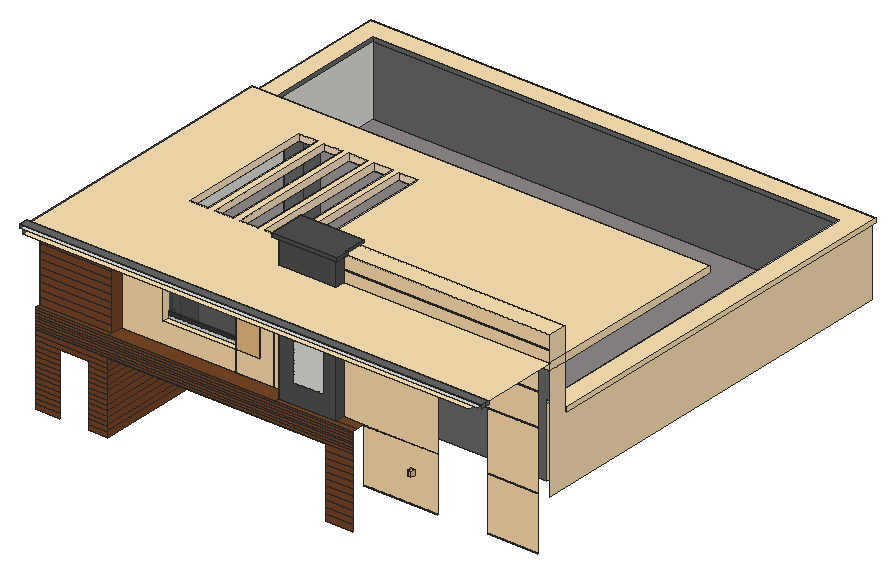
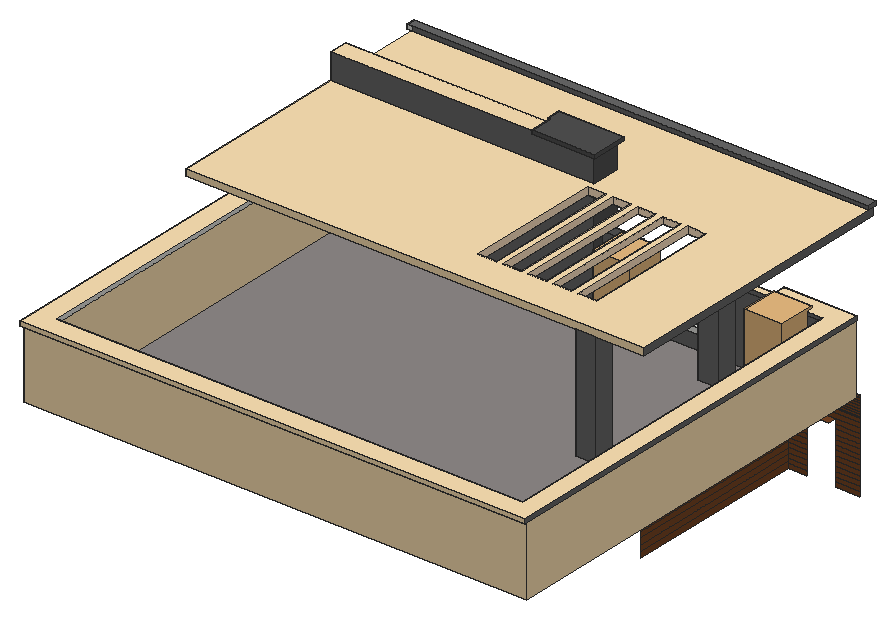
# SketchUp Ruby script. Lengths in inches.
U = 1.inch
M = Sketchup.active_model
def pt(a) = Geom::Point3d.new(a.map { |v| v * U })
def face(e, loops, mat)
  f = e.add_face(loops[0].map { |a| pt(a) })
  loops[1..].each { |l| e.add_face(l.map { |a| pt(a) }).erase! }
  f.material = f.back_material = mat if mat
  f
end
# faces: each face lists its corners as indices into pts; further lists are holes
def faces(e, pts, list, mat = nil) = list.each { |f| face(e, (f[0].is_a?(Array) ? f : [f]).map { |l| l.map { |i| pts[i] } }, mat) }
# xy, xz, yz: faces in a plane at the given z, y or x. An outline is a flat list of corners, or four numbers for a rectangle; further outlines are holes
def ring(l) = l.size == 4 ? [[l[0], l[1]], [l[2], l[1]], [l[2], l[3]], [l[0], l[3]]] : l.each_slice(2).to_a
def flat(e, list, mat, &to3) = list.each { |f| face(e, (f[0].is_a?(Array) ? f : [f]).map { |l| ring(l).map { |u, v| to3.(u, v) } }, mat) }
def xy(e, z, list, mat = nil) = flat(e, list, mat) { |x, y| [x, y, z] }
def xz(e, y, list, mat = nil) = flat(e, list, mat) { |x, z| [x, y, z] }
def yz(e, x, list, mat = nil) = flat(e, list, mat) { |y, z| [x, y, z] }
def lines(e, pts, list) = list.each { |a, b| e.add_line(pt(pts[a]), pt(pts[b])) }
# prism: a flat outline (further loops are holes) pulled along v
def prism(e, loops, v, mat = nil)
  f = face(e, loops, mat); d = Geom::Vector3d.new(v.map { |x| x * U })
  f.pushpull(f.normal.samedirection?(d) ? d.length : -d.length)
end
def box(e, o, s, mat = nil) = prism(e, [[o, [o[0] + s[0], o[1], o[2]], [o[0] + s[0], o[1] + s[1], o[2]], [o[0], o[1] + s[1], o[2]]]], [0, 0, s[2]], mat)
def at(x, y, z, deg = 0) = Geom::Transformation.translation(pt([x, y, z])) * Geom::Transformation.rotation(ORIGIN, Z_AXIS, deg.degrees)
def axes(o, x, y, z) = Geom::Transformation.new([*x, 0, *y, 0, *z, 0, *pt(o).to_a, 1])
def part(name) = M.definitions.add(name)
# library, detail: a bought-in or finely detailed component or shape, given as its bounding box
def library(name, o, s) = part(name).tap { |d| box(d.entities, o, s) }
def detail(e, o, s) = box(e.add_group.entities, o, s)
def put(e, d, t, mat = nil) = e.add_instance(d, t).tap { |i| i.material = mat if mat }
def group(e, t, mat = nil) = e.add_group.tap { |g| g.transformation = t; g.material = mat if mat }.entities
root = M.entities
M.materials.add("KORKULUK CAMI").color = [72, 76, 73]
M.materials["KORKULUK CAMI"].alpha = 0.5
M.materials.add("KORKULUK PROFİL").color = [58, 58, 58]
M.materials.add("[0012_Bisque]").color = [255, 228, 196]
M.materials.add("[0032_Moccasin]").color = [255, 228, 181]
M.materials.add("[0033_NavajoWhite]").color = [255, 222, 173]
M.materials.add("[0134_DimGray]").color = [105, 105, 105]
M.materials.add("[0135_DarkGray]").color = [81, 81, 81]
M.materials.add("[Stone Marble]").color = [143, 138, 136]
M.materials.add("[Wood Veneer 01]").color = [120, 70, 37]
c1 = library("Lamp Wall Outdoor 94-02",[-1.89,-4.65,-3.17],[3.78,4.65,6.35])
c2 = library("plant",[-22.43,-22.29,0],[44.86,44.58,89.56])
c3 = part("CAM KORKULUK")
g1 = group(c3.entities,at(15.11,0,0))
g2 = group(g1,at(31.92,0.79,0),"KORKULUK CAMI")
xy(g2,3.9375,[[-46.24,0,19.11,0.39],[-46.24,0.39,-45.85,7.09],[18.72,0.39,19.11,7.09]])
xy(g2,35.43,[[-46.24,0,19.11,0.39],[-46.24,0.39,-45.85,7.09],[18.72,0.39,19.11,7.09]])
xz(g2,0,[[-46.24,3.9375,19.11,35.43]])
xz(g2,0.39,[[-46.24,3.9375,-45.85,35.43],[-45.85,3.9375,18.72,35.43],[18.72,3.9375,19.11,35.43]])
xz(g2,7.09,[[-46.24,3.9375,-45.85,35.43],[18.72,3.9375,19.11,35.43]])
yz(g2,-46.24,[[0,3.9375,0.39,35.43],[0.39,3.9375,7.09,35.43]])
yz(g2,-45.85,[[0.39,3.9375,7.09,35.43]])
yz(g2,18.72,[[0.39,3.9375,7.09,35.43]])
yz(g2,19.11,[[0,3.9375,0.39,35.43],[0.39,3.9375,7.09,35.43]])
g3 = group(g1,at(95.77,0,0),"KORKULUK PROFİL")
prism(g3,[[[-110.875,0,0],[-110.875,7.875,0],[-108.91,7.875,0],[-108.91,1.97,0],[-45.91,1.97,0],[-45.91,7.875,0],[-43.95,7.875,0],[-43.95,0,0]]],[0,0,3.9375])
g4 = group(g1,at(95.77,0.39,35.43))
prism(g4,[[[-110.48,0,0],[-110.48,7.48,0],[-109.3,7.48,0],[-109.3,1.18,0],[-45.52,1.18,0],[-45.52,7.48,0],[-44.34,7.48,0],[-44.34,0,0]]],[0,0,0.79],"KORKULUK PROFİL")
g5 = group(c3.entities,at(0,0,-7.875))
box(g5,[0,0,0],[66.93,7.875,7.875])
c4 = library("Tlon Light 950 Ceiling 152 008",[-18.7,-18.7,-3.78],[37.4,37.4,3.56])
xy(root,219.625,[[1583.17,528.0625,1636.42,600.9375],[1636.42,528.0625,1668.92,600.9375]])
xy(root,221.7,[[1460.375,309.8125,1494.3,320.75]],"[Wood Veneer 01]")
xy(root,233,[[1518,309.8125,1518,528.0625,1777.8125,528.0625,1777.8125,330.25,1674.625,330.25,1674.625,319.48,1681.5,319.48,1681.5,319.875,1688.38,319.875,1688.38,319.48,1695.26,319.48,1695.26,319.875,1702.14,319.875,1702.14,319.48,1709.02,319.48,1709.02,319.875,1715.9,319.875,1715.9,319.48,1722.78,319.48,1722.78,319.875,1729.66,319.875,1729.66,319.48,1736.54,319.48,1736.54,319.875,1743.42,319.875,1743.42,319.48,1750.3,319.48,1750.3,319.875,1757.18,319.875,1757.18,319.48,1764.05,319.48,1764.05,319.875,1770.93,319.875,1770.93,319.48,1777.8125,319.48,1777.8125,309.8125]],"[Wood Veneer 01]")
xy(root,257,[[[1453.13,337.57,1717.17,337.57,1717.17,349.32,2009.5,349.32,2009.5,785.68,1453.13,785.68],[1542.22,541.15,1566.53,565.47],[1542.22,357.72,1566.53,382.03]]],"[Stone Marble]")
xy(root,257,[[1431.3125,309.8125,1518,315.75],[1518,309.8125,1717.17,329.6875],[1717.17,309.8125,1809.4375,315.75],[1784.8125,315.75,1809.4375,327.3125]],"[Wood Veneer 01]")
xy(root,281.625,[[1567.79,329.6875,1682.98,337.57]],"[0032_Moccasin]")
xy(root,326.75,[[1897.5625,327.3125,1957.25,348.375]])
xy(root,339.3125,[[1430.8125,315.25,1518,315.75],[1430.8125,315.75,1431.3125,809.9375],[1518,329.1875,1567.79,329.6875],[2031.3125,349.32,2033.75,807.5],[1431.3125,807.5,2033.75,809.9375]])
xy(root,339.3125,[[1677.98,324.6875,1717.17,329.6875],[1677.98,329.6875,1682.98,337.57]],"[0135_DarkGray]")
xy(root,344.3125,[[1430.8125,315.25,1518,315.25,1518,329.1875,1567.79,329.1875,1567.79,337.57,1453.13,337.57,1453.13,785.68,2009.5,785.68,2009.5,349.32,2033.75,349.32,2033.75,809.9375,1430.8125,809.9375]],"[0032_Moccasin]")
xy(root,344.3125,[[1677.98,324.6875,1717.17,337.57]],"[0135_DarkGray]")
xy(root,392.3125,[[2017.03,327.3125,2031.3125,327.5],[1542.22,357.72,1566.53,382.03],[1542.22,541.15,1566.53,565.47]])
xy(root,392.3125,[[1485.22,541.15,1542.22,565.47],[1566.53,541.15,2031.3125,565.47]],"[0012_Bisque]")
xy(root,392.3125,[[[1485.22,223.9375,1485.22,541.15,2031.3125,541.15,2031.3125,327.5,2017.03,327.5,2017.03,223.9375],[1576.06,358.48,1598.12,522.05],[1605.9,358.48,1627.96,522.05],[1635.75,358.48,1657.81,522.05],[1665.59,358.48,1687.65,522.05],[1695.43,358.48,1717.5,522.05],[1542.22,357.72,1566.53,382.03]]],"[0032_Moccasin]")
xy(root,400.3125,[[1485.22,218.9375,2031.3125,223.9375]])
xy(root,400.3125,[[[1485.22,228.9375,2031.3125,565.47],[1576.06,358.48,1598.12,522.05],[1605.9,358.48,1627.96,522.05],[1635.75,358.48,1657.81,522.05],[1665.59,358.48,1687.65,522.05],[1695.43,358.48,1717.5,522.05]]],"[0032_Moccasin]")
xy(root,405.3125,[[1485.22,218.9375,2036.3125,228.9375]],"[0134_DimGray]")
xy(root,430.75,[[1717.17,315.75,1717.17,349.32,1786.8125,349.32,1786.8125,327.3125,1784.8125,327.3125,1784.8125,315.75],[1784.8125,315.75,1789.8125,327.3125],[1786.8125,327.3125,1789.8125,327.5]])
xy(root,430.75,[[1789.8125,327.3125,2031.3125,327.3125,2031.3125,349.32,1786.8125,349.32,1786.8125,327.5,1789.8125,327.5]],"[0032_Moccasin]")
xy(root,430.75,[[1712.17,310.75,1789.8125,315.75],[1712.17,315.75,1717.17,354.32],[1717.17,349.32,1786.8125,354.32]],"[0135_DarkGray]")
xy(root,434.9375,[[1712.17,310.75,1789.8125,310.75,1789.8125,327.5,1786.8125,327.5,1786.8125,354.32,1712.17,354.32]],"[0135_DarkGray]")
xz(root,228.9375,[[2031.3125,400.3125,2036.3125,405.3125]])
xz(root,228.9375,[[1485.22,400.3125,2031.3125,405.3125]],"[0134_DimGray]")
xz(root,309.8125,[[1431.3125,148.25,1460.375,153.9],[1494.3,148.25,1518,153.9],[1777.8125,150.13,1809.4375,157.67],[1431.3125,153.9,1460.375,159.55],[1494.3,153.9,1518,159.55],
  [1777.8125,157.67,1809.4375,165.2],[1431.3125,159.55,1460.375,165.2],[1494.3,159.55,1518,165.2],[1431.3125,165.2,1460.375,170.85],[1494.3,165.2,1518,170.85],
  [1777.8125,165.2,1809.4375,172.73],[1431.3125,170.85,1460.375,176.5],[1494.3,170.85,1518,176.5],[1777.8125,172.73,1809.4375,180.27],[1431.3125,176.5,1460.375,182.15],
  [1494.3,176.5,1518,182.15],[1777.8125,180.27,1809.4375,187.8],[1431.3125,182.15,1460.375,187.8],[1494.3,182.15,1518,187.8],[1431.3125,187.8,1460.375,193.45],
  [1494.3,187.8,1518,193.45],[1777.8125,187.8,1809.4375,195.33],[1431.3125,193.45,1460.375,199.1],[1494.3,193.45,1518,199.1],[1777.8125,195.33,1809.4375,202.87],
  [1431.3125,199.1,1460.375,204.75],[1494.3,199.1,1518,204.75],[1777.8125,202.87,1809.4375,210.4],[1431.3125,204.75,1460.375,210.4],[1494.3,204.75,1518,210.4],
  [1431.3125,210.4,1460.375,216.05],[1494.3,210.4,1518,216.05],[1777.8125,210.4,1809.4375,217.93],[1431.3125,216.05,1460.375,221.7],[1494.3,216.05,1518,221.7],
  [1777.8125,217.93,1809.4375,225.47],[1431.3125,221.7,1518,227.35],[1777.8125,225.47,1809.4375,225.47,1809.4375,233.625,1431.3125,233.625,1431.3125,233,1777.8125,233],[1431.3125,227.35,1518,233],[1431.3125,233.625,1809.4375,236.55],
  [1431.3125,236.55,1809.4375,239.47],[1431.3125,239.47,1809.4375,242.39],[1431.3125,242.39,1809.4375,245.3125],[1431.3125,245.3125,1809.4375,248.23],[1431.3125,248.23,1809.4375,251.16],
  [1431.3125,251.16,1809.4375,254.08],[1431.3125,254.08,1809.4375,257]],"[Wood Veneer 01]")
xz(root,310.75,[[1712.17,430.75,1789.8125,434.9375]],"[0135_DarkGray]")
xz(root,315.25,[[1430.8125,339.3125,1518,344.3125]],"[0135_DarkGray]")
xz(root,315.75,[[1734.84,280.12,1768.77,347.56]])
xz(root,315.75,[[[1717.17,257,1784.8125,430.75],[1734.84,280.12,1768.77,347.56]]],"[0135_DarkGray]")
xz(root,315.75,[[1431.3125,257,1518,265.23],[1431.3125,265.23,1518,273.46],[1431.3125,273.46,1518,281.69],[1431.3125,281.69,1518,289.92],[1431.3125,289.92,1518,298.16],
  [1431.3125,298.16,1518,306.39],[1431.3125,306.39,1518,314.62],[1431.3125,314.62,1518,322.85],[1431.3125,322.85,1518,331.08],[1431.3125,331.08,1518,339.3125]],"[Wood Veneer 01]")
xz(root,324.6875,[[1677.98,339.3125,1717.17,344.3125]],"[0135_DarkGray]")
xz(root,327.3125,[[1809.4375,192.7,1897.5625,255.9375],[1957.25,192.7,2017.03,255.9375],[1809.4375,256.9375,1897.5625,256.9375,1897.5625,325.75,1784.8125,325.75,1784.8125,257,1809.4375,257],[1957.25,256.9375,2017.03,325.75],[1784.8125,326.75,2017.03,364.83],
  [1784.8125,365.83,2017.03,365.83,2017.03,392.3125,2031.3125,392.3125,2031.3125,413.25,1784.8125,413.25],[1784.8125,414.25,2031.3125,430.75]],"[0033_NavajoWhite]")
xz(root,327.3125,[[1809.4375,191.7,1897.5625,192.7],[1957.25,191.7,2017.03,192.7],[1809.4375,255.9375,1897.5625,256.9375],[1957.25,255.9375,2017.03,256.9375],[1784.8125,325.75,1897.5625,326.75],
  [1957.25,325.75,2017.03,326.75],[1784.8125,364.83,2017.03,365.83],[1784.8125,413.25,2031.3125,414.25]],"[0135_DarkGray]")
xz(root,327.5,[[1786.8125,430.75,1789.8125,434.9375]])
xz(root,329.1875,[[1518,339.3125,1567.79,344.3125]],"[0135_DarkGray]")
xz(root,329.6875,[[1518,257,1717.17,257,1717.17,339.3125,1682.98,339.3125,1682.98,281.625,1567.79,281.625,1567.79,339.3125,1518,339.3125]],"[0033_NavajoWhite]")
xz(root,337.57,[[1453.13,257,1453.13,339.3125,1567.79,339.3125,1567.79,281.625,1682.98,281.625,1682.98,339.3125,1677.98,339.3125,1677.98,344.3125,1717.17,344.3125,1717.17,257],[1453.13,339.3125,1567.79,344.3125]],"[0134_DimGray]")
xz(root,349.32,[[2031.3125,339.3125,2033.75,344.3125]])
xz(root,349.32,[[1717.17,257,1717.17,430.75,2031.3125,430.75,2031.3125,344.3125,2009.5,344.3125,2009.5,257]],"[0134_DimGray]")
xz(root,354.32,[[1712.17,430.75,1786.8125,434.9375]],"[0135_DarkGray]")
xz(root,357.72,[[1542.22,257,1566.53,392.3125]],"[0134_DimGray]")
xz(root,358.48,[[1576.06,392.3125,1598.12,400.3125],[1605.9,392.3125,1627.96,400.3125],[1635.75,392.3125,1657.81,400.3125],[1665.59,392.3125,1687.65,400.3125],[1695.43,392.3125,1717.5,400.3125]],"[0012_Bisque]")
xz(root,382.03,[[1542.22,257,1566.53,392.3125]],"[0134_DimGray]")
xz(root,522.05,[[1576.06,392.3125,1598.12,400.3125],[1605.9,392.3125,1627.96,400.3125],[1635.75,392.3125,1657.81,400.3125],[1665.59,392.3125,1687.65,400.3125],[1695.43,392.3125,1717.5,400.3125]],"[0012_Bisque]")
xz(root,541.15,[[1542.22,257,1566.53,392.3125]],"[0134_DimGray]")
xz(root,565.47,[[1485.22,392.3125,2031.3125,400.3125]],"[0032_Moccasin]")
xz(root,565.47,[[1542.22,257,1566.53,392.3125]],"[0134_DimGray]")
xz(root,785.68,[[1453.13,257,2009.5,339.3125],[1453.13,339.3125,2009.5,344.3125]],"[0134_DimGray]")
xz(root,807.5,[[1431.3125,257,2031.3125,339.3125]],"[0032_Moccasin]")
xz(root,809.9375,[[1430.8125,339.3125,2033.75,344.3125]],"[0032_Moccasin]")
yz(root,1430.8125,[[315.25,339.3125,809.9375,344.3125]],"[0134_DimGray]")
yz(root,1431.3125,[[315.75,257,807.5,339.3125]],"[0032_Moccasin]")
yz(root,1453.13,[[337.57,257,785.68,339.3125]])
yz(root,1453.13,[[337.57,339.3125,785.68,344.3125]],"[0134_DimGray]")
yz(root,1485.22,[[223.9375,392.3125,565.47,400.3125],[218.9375,400.3125,228.9375,405.3125]],"[0134_DimGray]")
yz(root,1518,[[315.25,339.3125,329.1875,344.3125]],"[0135_DarkGray]")
yz(root,1518,[[309.8125,148.2,528.0625,155.27],[309.8125,155.27,528.0625,162.33],[309.8125,162.33,528.0625,169.4],[309.8125,169.4,528.0625,176.47],[309.8125,176.47,528.0625,183.53],
  [309.8125,183.53,528.0625,190.6],[309.8125,190.6,528.0625,197.67],[309.8125,197.67,528.0625,204.73],[309.8125,204.73,528.0625,211.8],[309.8125,211.8,528.0625,218.87],
  [309.8125,218.87,528.0625,225.93],[309.8125,225.93,528.0625,233],[315.75,257,329.6875,339.3125]],"[Wood Veneer 01]")
yz(root,1542.22,[[357.72,257,382.03,392.3125],[541.15,257,565.47,392.3125]],"[0134_DimGray]")
yz(root,1566.53,[[357.72,257,382.03,392.3125],[541.15,257,565.47,392.3125]],"[0134_DimGray]")
yz(root,1567.79,[[329.6875,281.625,337.57,339.3125]],"[0032_Moccasin]")
yz(root,1567.79,[[329.1875,339.3125,337.57,344.3125]],"[0135_DarkGray]")
yz(root,1576.06,[[358.48,392.3125,522.05,400.3125]],"[0012_Bisque]")
yz(root,1598.12,[[358.48,392.3125,522.05,400.3125]],"[0012_Bisque]")
yz(root,1605.9,[[358.48,392.3125,522.05,400.3125]],"[0012_Bisque]")
yz(root,1627.96,[[358.48,392.3125,522.05,400.3125]],"[0012_Bisque]")
yz(root,1635.75,[[358.48,392.3125,522.05,400.3125]],"[0012_Bisque]")
yz(root,1657.81,[[358.48,392.3125,522.05,400.3125]],"[0012_Bisque]")
yz(root,1665.59,[[358.48,392.3125,522.05,400.3125]],"[0012_Bisque]")
yz(root,1677.98,[[324.6875,339.3125,337.57,344.3125]],"[0135_DarkGray]")
yz(root,1682.98,[[329.6875,281.625,337.57,339.3125]],"[0032_Moccasin]")
yz(root,1687.65,[[358.48,392.3125,522.05,400.3125]],"[0012_Bisque]")
yz(root,1695.43,[[358.48,392.3125,522.05,400.3125]],"[0012_Bisque]")
yz(root,1712.17,[[310.75,430.75,354.32,434.9375]],"[0135_DarkGray]")
yz(root,1717.17,[[315.75,257,329.6875,339.3125]],"[0032_Moccasin]")
yz(root,1717.17,[[337.57,257,337.57,344.3125,324.6875,344.3125,324.6875,339.3125,315.75,339.3125,315.75,430.75,349.32,430.75,349.32,257]],"[0135_DarkGray]")
yz(root,1717.5,[[358.48,392.3125,522.05,400.3125]],"[0012_Bisque]")
yz(root,1784.8125,[[315.75,257,327.3125,430.75]],"[0135_DarkGray]")
yz(root,1786.8125,[[327.5,430.75,354.32,434.9375]],"[0135_DarkGray]")
yz(root,1789.8125,[[310.75,430.75,327.5,434.9375]],"[0135_DarkGray]")
yz(root,2009.5,[[349.32,339.3125,785.68,344.3125]])
yz(root,2009.5,[[349.32,257,785.68,339.3125]],"[0032_Moccasin]")
yz(root,2031.3125,[[327.5,257,807.5,257,807.5,339.3125,349.32,339.3125,349.32,392.3125,327.5,392.3125],[327.3125,392.3125,349.32,400.3125],[349.32,392.3125,565.47,400.3125],[327.3125,400.3125,349.32,430.75]],"[0032_Moccasin]")
yz(root,2033.75,[[349.32,339.3125,809.9375,344.3125]],"[0032_Moccasin]")
yz(root,2036.3125,[[218.9375,400.3125,223.9375,405.3125],[223.9375,400.3125,228.9375,405.3125]],"[0134_DimGray]")
put(root,c1,at(1693.72,528.0625,194.2))
put(root,c1,at(1867.34,327.3125,226.63))
put(root,c2,at(1495.57,351.98,257))
put(root,c2,at(1676.76,351.98,257))
put(root,c3,axes([1565.24,337.06,285.41],[1.8404,0,0],[0,0.93154,0],[0,0,0.8983]))
put(root,c1,at(1755.34,315.75,361.6875))
put(root,c4,axes([1501.79,261.46,392.34],[0.12,0,0],[0,0.12,0],[0,0,0.12]))
put(root,c4,axes([1618.01,261.46,392.34],[0.12,0,0],[0,0.12,0],[0,0,0.12]))
put(root,c4,axes([1734.23,261.46,392.34],[0.12,0,0],[0,0.12,0],[0,0,0.12]))
put(root,c4,axes([1850.45,261.46,392.34],[0.12,0,0],[0,0.12,0],[0,0,0.12]))
put(root,c4,axes([1966.66,261.46,392.34],[0.12,0,0],[0,0.12,0],[0,0,0.12]))
